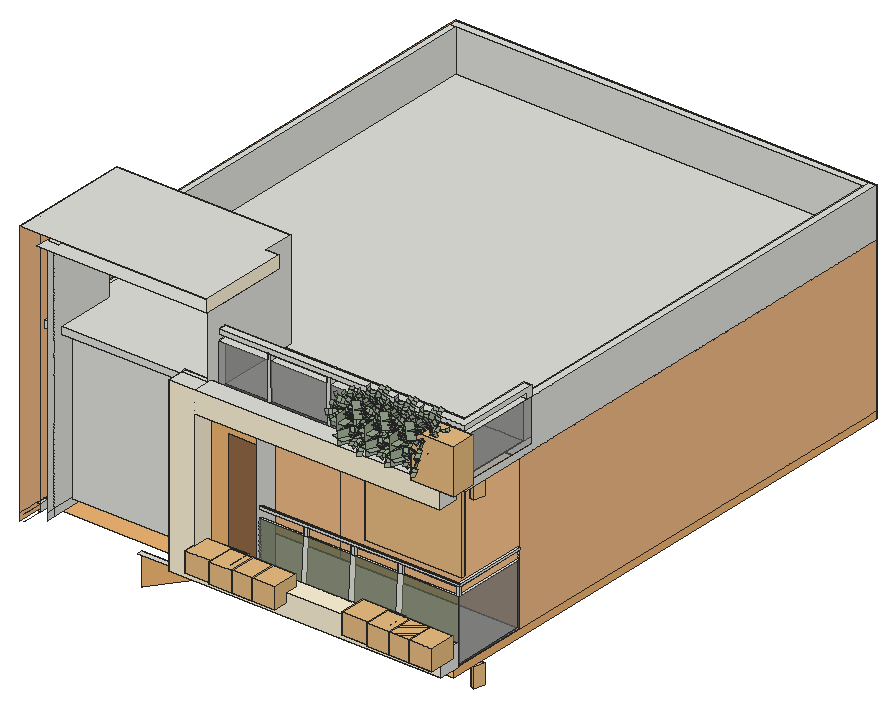
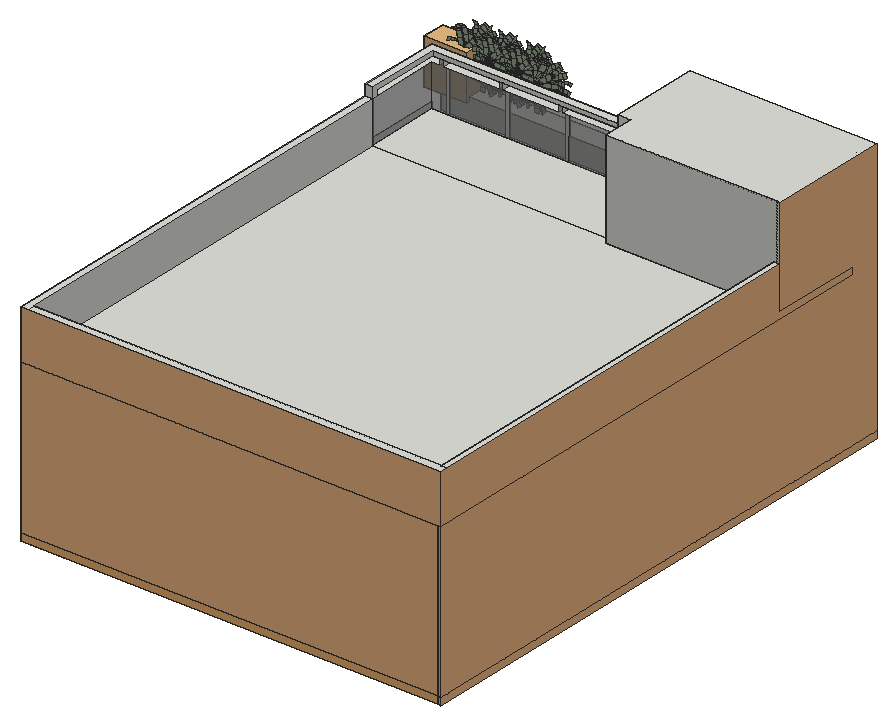
# SketchUp Ruby script. Lengths in inches.
U = 1.inch
M = Sketchup.active_model
def pt(a) = Geom::Point3d.new(a.map { |v| v * U })
def face(e, loops, mat)
  f = e.add_face(loops[0].map { |a| pt(a) })
  loops[1..].each { |l| e.add_face(l.map { |a| pt(a) }).erase! }
  f.material = f.back_material = mat if mat
  f
end
# faces: each face lists its corners as indices into pts; further lists are holes
def faces(e, pts, list, mat = nil) = list.each { |f| face(e, (f[0].is_a?(Array) ? f : [f]).map { |l| l.map { |i| pts[i] } }, mat) }
# xy, xz, yz: faces in a plane at the given z, y or x. An outline is a flat list of corners, or four numbers for a rectangle; further outlines are holes
def ring(l) = l.size == 4 ? [[l[0], l[1]], [l[2], l[1]], [l[2], l[3]], [l[0], l[3]]] : l.each_slice(2).to_a
def flat(e, list, mat, &to3) = list.each { |f| face(e, (f[0].is_a?(Array) ? f : [f]).map { |l| ring(l).map { |u, v| to3.(u, v) } }, mat) }
def xy(e, z, list, mat = nil) = flat(e, list, mat) { |x, y| [x, y, z] }
def xz(e, y, list, mat = nil) = flat(e, list, mat) { |x, z| [x, y, z] }
def yz(e, x, list, mat = nil) = flat(e, list, mat) { |y, z| [x, y, z] }
def lines(e, pts, list) = list.each { |a, b| e.add_line(pt(pts[a]), pt(pts[b])) }
# prism: a flat outline (further loops are holes) pulled along v
def prism(e, loops, v, mat = nil)
  f = face(e, loops, mat); d = Geom::Vector3d.new(v.map { |x| x * U })
  f.pushpull(f.normal.samedirection?(d) ? d.length : -d.length)
end
def box(e, o, s, mat = nil) = prism(e, [[o, [o[0] + s[0], o[1], o[2]], [o[0] + s[0], o[1] + s[1], o[2]], [o[0], o[1] + s[1], o[2]]]], [0, 0, s[2]], mat)
def at(x, y, z, deg = 0) = Geom::Transformation.translation(pt([x, y, z])) * Geom::Transformation.rotation(ORIGIN, Z_AXIS, deg.degrees)
def axes(o, x, y, z) = Geom::Transformation.new([*x, 0, *y, 0, *z, 0, *pt(o).to_a, 1])
def part(name) = M.definitions.add(name)
# library, detail: a bought-in or finely detailed component or shape, given as its bounding box
def library(name, o, s) = part(name).tap { |d| box(d.entities, o, s) }
def detail(e, o, s) = box(e.add_group.entities, o, s)
def put(e, d, t, mat = nil) = e.add_instance(d, t).tap { |i| i.material = mat if mat }
def group(e, t, mat = nil) = e.add_group.tap { |g| g.transformation = t; g.material = mat if mat }.entities
root = M.entities
M.materials.add("[Brick Antique 01]").color = [147, 105, 71]
M.materials.add("[Color C03]").color = [242, 183, 116]
M.materials.add("[Color C03]1").color = [242, 188, 135]
M.materials.add("[Color D01]").color = [255, 245, 216]
M.materials.add("[Translucent Glass Dark Green]").color = [62, 91, 5]
M.materials["[Translucent Glass Dark Green]"].alpha = 0.5
M.materials.add("[Translucent Glass Gray]").color = [128, 128, 128]
M.materials["[Translucent Glass Gray]"].alpha = 0.5
M.materials.add("hymenocallis littoralis").color = [156, 172, 146]
c1 = library("[SKP_VZ_MOD_01]_WALL_LIGHT",[-1.1,-1.22,0],[3.54,2.36,6.3])
c2 = library("Plante \#58",[-0.43,-1.58,0],[20.84,18.06,17.59])
c3 = part("Group\#4")
xy(c3.entities,35.0625,[[0,2,3.83,3.5]])
p = [[0,2,35.0625],[0,0,0],[3.83,0,0],[3.83,2,35.0625]]
faces(c3.entities,p,[[0,1,2,3]])
c4 = library("Group\#6",[0,0,0],[84,7.18,89.375])
c5 = part("Group\#856")
xy(c5.entities,7.38,[[0,0,5.5,15.91]],"hymenocallis littoralis")
p = [[5.5,28.78,0],[5.5,26.79,3.44],[0,26.79,3.44],[0,28.78,0],[0,23.75,6],[5.5,23.75,6],
  [0,15.91,7.38],[5.5,15.91,7.38]]
faces(c5.entities,p,[[0,1,2,3],[4,2,1,5],[6,4,5,7]],"hymenocallis littoralis")
c6 = part("Group\#12")
xy(c6.entities,7.38,[[0,0,5.5,15.91],[0,15.91,5.5,23.87]],"hymenocallis littoralis")
p = [[5.5,31.07,4.3],[5.5,27.74,6.47],[0,27.74,6.47],[0,31.07,4.3],[0,23.87,7.38],[5.5,23.87,7.38]]
faces(c6.entities,p,[[0,1,2,3],[4,2,1,5]],"hymenocallis littoralis")
c7 = part("Group\#857")
xy(c7.entities,7.38,[[0,0,5.6,15.91]],"hymenocallis littoralis")
p = [[5.6,28.78,0],[5.6,26.79,3.44],[0,26.79,3.44],[0,28.78,0],[0,23.75,6],[5.6,23.75,6],
  [0,15.91,7.38],[5.6,15.91,7.38]]
faces(c7.entities,p,[[0,1,2,3],[4,2,1,5],[6,4,5,7]],"hymenocallis littoralis")
c8 = part("Group\#855")
put(c8.entities,c6,axes([6.09,8.57,-0.52],[0.446,0.85617,0.26089],[-0.18444,-0.19731,0.96283],[0.87582,-0.47754,0.0699]))
put(c8.entities,c6,axes([6.29,7.28,-1.71],[0.37058,0.92707,-0.05667],[-0.32382,0.19004,0.99128],[0.87712,-0.32925,0.34964]))
put(c8.entities,c6,axes([11.04,16.14,-0.7],[1,0,0],[0,0.16628,1.02662],[0,-1.18456,0.19186]))
c9 = part("Group\#860")
put(c9.entities,c5,axes([24.57,32.05,-1.76],[0.9552,-0.22102,-0.19681],[0.4036,0.95545,0.88585],[-0.00568,-0.67859,0.7345]))
put(c9.entities,c5,axes([23.95,29.24,-2.4],[0,1,0],[-0.76041,0,0.64945],[0.64945,0,0.76041]))
put(c9.entities,c5,axes([24.22,24.72,-0.48],[-0.70711,0.70711,0],[-0.32757,-0.32757,0.80237],[0.61237,0.61237,0.5]))
put(c9.entities,c6,axes([20.66,37.22,-0.63],[1.12361,0.03262,0.39091],[-0.43499,0.29739,0.78777],[0.09852,-1.27434,0.37535]))
put(c9.entities,c5,axes([28.75,24.45,-2.4],[-1,0,0],[0,-0.76041,0.64945],[0,0.64945,0.76041]))
put(c9.entities,c7,axes([30.4,30.98,-3.7],[0.65676,-0.72002,0.22414],[0.55667,0.66341,0.5],[-0.50871,-0.20361,0.83652]))
put(c9.entities,c7,axes([32.41,29.61,-3.7],[0.04029,-0.97372,0.22414],[0.85287,0.15038,0.5],[-0.52057,0.17102,0.83652]))
put(c9.entities,c5,axes([31.89,25.85,-1.76],[-0.92056,0.33739,-0.19681],[-0.5186,-0.89824,0.88585],[0.08952,0.67268,0.7345]))
put(c9.entities,c5,axes([25.55,34.78,-0.48],[0.86603,0.5,0],[-0.25,0.43301,0.86603],[0.43301,-0.75,0.5]))
put(c9.entities,c7,axes([20.4,16.9375,-8.07],[-0.70711,0.70711,0],[-0.35754,-0.35754,0.65422],[1.3987,1.3987,1.52882]))
put(c9.entities,c5,axes([32.86,34.14,-0.48],[0.76604,-0.64279,0],[0.32139,0.38302,0.86603],[-0.55667,-0.66341,0.5]))
put(c9.entities,c5,axes([27.15,34.7,-0.1],[0.82472,-0.17528,-0.53769],[0.53769,0.53769,0.64945],[0.17528,-0.82472,0.53769]))
put(c9.entities,c5,axes([33.58,28.77,-2.4],[0,-1,0],[0.76041,0,0.64945],[-0.64945,0,0.76041]))
put(c9.entities,c5,axes([26.43,23.87,-2.81],[-0.75126,0.04415,0.65853],[0.53769,-0.53769,0.64945],[0.38276,0.84199,0.3802]))
put(c9.entities,c5,axes([28.78,23.98,-2.4],[-1,0,0],[0,-0.76041,0.64945],[0,0.64945,0.76041]))
put(c9.entities,c5,axes([25.39,25.38,-2.4],[-0.70711,0.70711,0],[-0.53769,-0.53769,0.64945],[0.45923,0.45923,0.76041]))
put(c9.entities,c5,axes([27.32,21.63,-0.1],[-0.45923,0.70711,-0.53769],[-0.76041,0,0.64945],[0.45923,0.70711,0.53769]))
put(c9.entities,c5,axes([25.17,27.625,-1.76],[0.56416,0.80187,-0.19681],[-0.66673,0.66673,0.80532],[0.62659,-0.26057,0.7345]))
put(c9.entities,c7,axes([27.59,27.04,-3.96],[-0.8993,-0.06127,0.43301],[0.2962,-0.8138,0.5],[0.32175,0.57791,0.75]))
put(c9.entities,c7,axes([26.98,24.5,-3.18],[-0.5,0.86603,0],[-0.75,-0.43301,0.5],[0.43301,0.25,0.86603]))
put(c9.entities,c7,axes([24.55,27.74,-3.7],[0.29517,0.92878,0.22414],[-0.85287,0.15038,0.5],[0.43068,-0.33875,0.83652]))
put(c9.entities,c7,axes([24.26,29.8,-3.18],[0.76604,0.64279,0],[-0.47317,0.5639,0.425],[0.32139,-0.38302,0.86603]))
put(c9.entities,c7,axes([25.98,32.46,-3.18],[1,0,0],[0,0.86603,0.5],[0,-0.5,0.86603]))
put(c9.entities,c5,axes([28.78,33.57,-2.4],[1,0,0],[0,0.76041,0.64945],[0,-0.64945,0.76041]))
put(c9.entities,c8,at(14.99,21.38,2.5))
put(c9.entities,c6,axes([34.63,26.34,-1.46],[-0.70089,-0.70877,0.07994],[0.4756,-0.38088,0.79293],[-0.53156,0.59378,0.60405]))
put(c9.entities,c6,axes([28.14,16.92,1.8125],[-1.19719,0.6912,0],[-0.09607,-0.16641,0.94244],[0.68444,1.18549,0.17613]))
put(c9.entities,c6,axes([31.5625,35.84,0.97],[0.66765,-1.1564,0.35779],[0.04445,0.30732,0.91033],[-1.20828,-0.64496,0.17012]))
put(c9.entities,c6,axes([38.94,22.51,0.89],[-0.97932,-0.67164,-0.05202],[0.27787,-0.41401,0.90999],[-0.85985,0.93577,0.32097]))
put(c9.entities,c6,axes([38.44,21.09,1.98],[-1.02864,-0.54856,0.2395],[0.33481,0.06999,0.88388],[-0.77261,1.08328,0.06417]))
put(c9.entities,c7,axes([35.02,30.51,-1.3],[-0.17365,-0.98481,0],[0.60224,-0.10619,0.79122],[-0.7792,0.13739,0.61153]))
put(c9.entities,c7,axes([29.41,22.33,-1.3],[-0.93969,0.34202,0],[-0.20915,-0.57465,0.79122],[0.27061,0.74351,0.61153]))
put(c9.entities,c6,axes([19.64,36,-1.62],[1.18194,0.09546,0.08234],[-0.14377,0.68823,0.76313],[0.21457,-1.1326,0.62386]))
put(c9.entities,c7,axes([24.25,24.14,-1.3],[-0.34202,0.93969,0],[-0.57465,-0.20915,0.79122],[0.74351,0.27061,0.61153]))
put(c9.entities,c7,axes([25.98,34.61,-1.3],[1,0,0],[0,0.61153,0.79122],[0,-0.79122,0.61153]))
put(c9.entities,c7,axes([31.16,34.41,-1.64],[0.56518,-0.80224,-0.19234],[0.73413,0.34233,0.72935],[-0.47639,-0.50772,0.71782]))
put(c9.entities,c7,axes([40.52,26.84,-5.82],[-0.42262,-0.90631,0],[0.48019,-0.22391,0.68552],[-1.43418,0.66877,1.22305]))
put(c9.entities,c5,axes([29.86,38.42,-1.01],[0.89064,-0.37013,0.26413],[-0.03924,0.63286,1.01918],[-0.45353,-0.76487,0.45748]))
put(c9.entities,c5,axes([29.34,22.4,-0.48],[-0.99619,-0.08716,0],[0.04358,-0.4981,0.86603],[-0.07548,0.86273,0.5]))
c10 = part("Group\#859")
put(c10.entities,c5,axes([24.57,32.05,-1.76],[0.9552,-0.22102,-0.19681],[0.4036,0.95545,0.88585],[-0.00568,-0.67859,0.7345]))
put(c10.entities,c5,axes([23.95,29.24,-2.4],[0,1,0],[-0.76041,0,0.64945],[0.64945,0,0.76041]))
put(c10.entities,c5,axes([24.22,24.72,-0.48],[-0.70711,0.70711,0],[-0.32757,-0.32757,0.80237],[0.61237,0.61237,0.5]))
put(c10.entities,c6,axes([22.87,39.97,-0.63],[1.12361,0.03262,0.39091],[-0.43499,0.29739,0.78777],[0.09852,-1.27434,0.37535]))
put(c10.entities,c5,axes([28.75,24.45,-2.4],[-1,0,0],[0,-0.76041,0.64945],[0,0.64945,0.76041]))
put(c10.entities,c7,axes([30.4,30.98,-3.7],[0.65676,-0.72002,0.22414],[0.55667,0.66341,0.5],[-0.50871,-0.20361,0.83652]))
put(c10.entities,c7,axes([32.41,29.61,-3.7],[0.04029,-0.97372,0.22414],[0.85287,0.15038,0.5],[-0.52057,0.17102,0.83652]))
put(c10.entities,c5,axes([31.89,25.85,-1.76],[-0.92056,0.33739,-0.19681],[-0.5186,-0.89824,0.88585],[0.08952,0.67268,0.7345]))
put(c10.entities,c5,axes([25.55,34.78,-0.48],[0.86603,0.5,0],[-0.25,0.43301,0.86603],[0.43301,-0.75,0.5]))
put(c10.entities,c7,axes([20.4,16.9375,-8.07],[-0.70711,0.70711,0],[-0.35754,-0.35754,0.65422],[1.3987,1.3987,1.52882]))
put(c10.entities,c5,axes([32.86,34.14,-0.48],[0.76604,-0.64279,0],[0.32139,0.38302,0.86603],[-0.55667,-0.66341,0.5]))
put(c10.entities,c5,axes([27.15,34.7,-0.1],[0.82472,-0.17528,-0.53769],[0.53769,0.53769,0.64945],[0.17528,-0.82472,0.53769]))
put(c10.entities,c5,axes([33.58,28.77,-2.4],[0,-1,0],[0.76041,0,0.64945],[-0.64945,0,0.76041]))
put(c10.entities,c5,axes([26.43,23.87,-2.81],[-0.75126,0.04415,0.65853],[0.53769,-0.53769,0.64945],[0.38276,0.84199,0.3802]))
put(c10.entities,c5,axes([28.78,23.98,-2.4],[-1,0,0],[0,-0.76041,0.64945],[0,0.64945,0.76041]))
put(c10.entities,c5,axes([25.39,25.38,-2.4],[-0.70711,0.70711,0],[-0.53769,-0.53769,0.64945],[0.45923,0.45923,0.76041]))
put(c10.entities,c5,axes([27.32,21.63,-0.1],[-0.45923,0.70711,-0.53769],[-0.76041,0,0.64945],[0.45923,0.70711,0.53769]))
put(c10.entities,c5,axes([25.17,27.625,-1.76],[0.56416,0.80187,-0.19681],[-0.66673,0.66673,0.80532],[0.62659,-0.26057,0.7345]))
put(c10.entities,c7,axes([27.59,27.04,-3.96],[-0.8993,-0.06127,0.43301],[0.2962,-0.8138,0.5],[0.32175,0.57791,0.75]))
put(c10.entities,c7,axes([33.07,28.9375,-1.86],[-0.5,0.86603,0],[-0.86347,-0.49852,0.1661],[0.11853,0.06843,0.98016]))
put(c10.entities,c7,axes([24.55,27.74,-3.7],[0.29517,0.92878,0.22414],[-0.85287,0.15038,0.5],[0.43068,-0.33875,0.83652]))
put(c10.entities,c7,axes([24.26,29.8,-3.18],[0.76604,0.64279,0],[-0.47317,0.5639,0.425],[0.32139,-0.38302,0.86603]))
put(c10.entities,c7,axes([25.98,32.46,-3.18],[1,0,0],[0,0.86603,0.5],[0,-0.5,0.86603]))
put(c10.entities,c5,axes([28.78,33.57,-2.4],[1,0,0],[0,0.76041,0.64945],[0,-0.64945,0.76041]))
put(c10.entities,c8,at(14.99,21.38,2.5))
put(c10.entities,c6,axes([34.63,26.34,-1.46],[-0.70089,-0.70877,0.07994],[0.4756,-0.38088,0.79293],[-0.53156,0.59378,0.60405]))
put(c10.entities,c6,axes([28.14,16.92,1.8125],[-1.19719,0.6912,0],[-0.09607,-0.16641,0.94244],[0.68444,1.18549,0.17613]))
put(c10.entities,c6,axes([31.5625,35.84,0.97],[0.66765,-1.1564,0.35779],[0.04445,0.30732,0.91033],[-1.20828,-0.64496,0.17012]))
put(c10.entities,c6,axes([38.94,22.51,0.89],[-0.97932,-0.67164,-0.05202],[0.27787,-0.41401,0.90999],[-0.85985,0.93577,0.32097]))
put(c10.entities,c6,axes([38.44,21.09,1.98],[-1.02864,-0.54856,0.2395],[0.33481,0.06999,0.88388],[-0.77261,1.08328,0.06417]))
put(c10.entities,c7,axes([35.02,30.51,-1.3],[-0.17365,-0.98481,0],[0.60224,-0.10619,0.79122],[-0.7792,0.13739,0.61153]))
put(c10.entities,c7,axes([29.41,22.33,-1.3],[-0.93969,0.34202,0],[-0.20915,-0.57465,0.79122],[0.27061,0.74351,0.61153]))
put(c10.entities,c6,axes([19.64,36,-1.62],[1.18194,0.09546,0.08234],[-0.14377,0.68823,0.76313],[0.21457,-1.1326,0.62386]))
put(c10.entities,c7,axes([24.25,24.14,-1.3],[-0.34202,0.93969,0],[-0.57465,-0.20915,0.79122],[0.74351,0.27061,0.61153]))
put(c10.entities,c7,axes([25.98,34.61,-1.3],[1,0,0],[0,0.61153,0.79122],[0,-0.79122,0.61153]))
put(c10.entities,c7,axes([31.16,34.41,-1.64],[0.56518,-0.80224,-0.19234],[0.73413,0.34233,0.72935],[-0.47639,-0.50772,0.71782]))
put(c10.entities,c7,axes([40.52,26.84,-5.82],[-0.42262,-0.90631,0],[0.48019,-0.22391,0.68552],[-1.43418,0.66877,1.22305]))
put(c10.entities,c5,axes([29.86,38.42,-1.01],[0.89064,-0.37013,0.26413],[-0.03924,0.63286,1.01918],[-0.45353,-0.76487,0.45748]))
put(c10.entities,c5,axes([29.34,22.4,-0.48],[-0.99619,-0.08716,0],[0.04358,-0.4981,0.86603],[-0.07548,0.86273,0.5]))
put(c10.entities,c7,axes([25.22,28.39,-0.16],[0.48481,0.87462,0],[-0.87203,0.48338,0.1661],[0.11971,-0.06635,0.98016]))
put(c10.entities,c7,axes([24.56,24.29,-4.78],[0.48481,0.87462,0],[-0.87203,0.48338,0.1661],[0.11971,-0.06635,0.98016]))
put(c10.entities,c7,axes([23.9375,27.06,-4.78],[0.99753,0.07018,0],[-0.06998,0.99459,0.1661],[0.00961,-0.13653,0.98016]))
put(c10.entities,c7,axes([25.92,29.09,-4.78],[0.6025,-0.79812,0],[0.79576,0.60072,0.1661],[-0.10924,-0.08246,0.98016]))
put(c10.entities,c7,axes([28.7,28.53,-4.78],[-0.34082,-0.94013,0],[0.93735,-0.33981,0.1661],[-0.12867,0.04665,0.98016]))
c11 = part("Group\#858")
xz(c11.entities,10.07,[[9.07,0,10.07,31.01],[0,31.01,0,45.12,20.13,45.12,20.13,31.01,10.07,31.01,10.07,32.58,9.07,32.58,9.07,31.01]],"hymenocallis littoralis")
yz(c11.entities,10.07,[[0,31.01,20.13,45.12]],"hymenocallis littoralis")
p = [[9.57,9.2,0],[10.07,10.07,0],[10.07,10.07,31.01],[10.07,10.07,32.58],[9.57,9.2,32.58]]
faces(c11.entities,p,[[0,1,2,3,4]],"hymenocallis littoralis")
c12 = part("cây lá nắng")
put(c12.entities,c9,axes([49.26,-2.75,0],[0.63109,0.63109,0],[-0.63109,0.63109,0],[0,0,0.935]))
put(c12.entities,c10,axes([26.6,-8.68,0],[0.63109,0.63109,0],[-0.63109,0.63109,0],[0,0,0.935]))
put(c12.entities,c11,axes([29.71,14.29,6.94],[0.425,0.73612,0],[-0.6771,0.39092,-0.33349],[-0.26859,0.15507,0.72712]))
put(c12.entities,c11,axes([42.0625,26.12,6.94],[0.85,0,0],[0,0.78185,-0.33349],[0,0.33349,0.78185]))
put(c12.entities,c9,axes([7.3125,23.0625,0],[0.8925,0,0],[0,0.8925,0],[0,0,0.935]))
put(c12.entities,c11,axes([24.4375,40.23,2.05],[0.85,0,0],[0,0.85,0],[0,0,0.85]))
c13 = part("Planting+101")
put(c13.entities,c12,axes([21.34,32.96,-4.59],[0,-0.71,0],[-0.71,0,0],[0,0,0.71]))
xy(root,114,[[196.3125,117.47,241.3125,128.9],[280.3125,117.47,364.3125,146.78]])
xy(root,138,[[139.52,45.9,196.3125,50.65],[196.3125,45.9,199.52,50.65],[49.3125,49.9,52.3125,59.47],[196.3125,50.65,199.52,59.47],[49.3125,59.47,52.3125,109.47],
  [49.3125,109.47,52.3125,117.47],[49.3125,117.47,52.3125,501.47],[52.3125,117.47,412.3125,501.47]])
xy(root,138,[[199.52,45.9,199.52,59.47,196.3125,59.47,196.3125,117.47,256.62,117.47,256.62,45.9],[[256.62,45.9,412.3125,117.47],[399.28,70.78,410.47,80.47]],[52.3125,59.47,196.3125,117.47]],"[Color C03]")
xy(root,144,[[177.125,31.9,412.3125,45.9],[177.125,45.9,199.52,49.9],[199.52,45.9,239.27,49.9],[239.27,45.9,412.3125,49.9],[49.3125,49.9,52.3125,57.47],
  [239.27,49.9,412.3125,51.9],[239.27,51.9,412.3125,53.4],[239.27,53.4,410.25,53.4,410.25,117.47,52.3125,117.47,52.3125,68.97,239.27,68.97],[410.25,53.4,412.3125,117.47],[49.3125,57.47,52.3125,109.47],
  [49.3125,109.47,52.3125,117.47],[49.3125,117.47,52.3125,501.47],[52.3125,117.47,412.3125,501.47]])
xy(root,162.75,[[199.52,31.9,412.3125,49.9]],"[Color D01]")
xy(root,168,[[280.3125,117.47,364.3125,133.97]])
xy(root,197.8125,[[239.27,51.9,277.74,53.4],[277.74,51.9,281.49,53.4],[281.49,51.9,281.57,53.4],[281.57,51.9,318.55,53.4],[318.55,51.9,322.38,53.4],
  [322.38,51.9,359.36,53.4],[359.36,51.9,363.19,53.4],[363.19,51.9,410.25,53.4],[410.25,53.53,412.3125,117.47]])
xy(root,205,[[239.27,51.9,277.74,53.4],[277.74,51.9,281.49,53.4],[281.49,51.9,318.55,53.4],[318.55,51.9,322.38,53.4],[322.38,51.9,359.36,53.4],
  [359.36,51.9,363.19,53.4],[363.19,51.9,410.25,53.4],[410.25,53.53,412.3125,117.47]])
xy(root,207,[[239.27,51.9,412.3125,53.4],[410.25,53.4,412.3125,117.47]])
xy(root,252,[[280.3125,117.47,364.3125,133.97]])
xy(root,273.03,[[199.52,31.9,410.875,49.9]],"[Color D01]")
xy(root,276,[[199.52,49.9,239.27,57.47],[49.3125,57.47,52.3125,68.97],[52.3125,57.47,196.3125,68.97],[196.3125,57.47,196.3125,68.97,239.27,68.97,239.27,57.9,199.52,57.9,199.52,57.47],[199.52,57.47,239.27,57.9],
  [49.3125,68.97,52.3125,109.47],[52.3125,68.97,196.3125,117.47],[49.3125,109.47,52.3125,117.47],[49.3125,117.47,52.3125,501.47]])
xy(root,276,[[239.27,57.9,239.27,68.97,196.3125,68.97,196.3125,117.47,256.62,117.47,256.62,57.9],[256.62,57.9,412.3125,117.47]],"[Color D01]")
xy(root,282,[[49.3125,57.47,52.3125,135.65],[52.3125,57.47,196.3125,135.65],[196.3125,57.47,199.52,129.47],[199.52,65.22,405.9375,129.47],[199.52,129.47,405.9375,129.47,405.9375,494.53,54.75,494.53,54.75,135.65,199.52,135.65],
  [196.3125,129.47,199.52,135.65]])
xy(root,291.78,[[177.125,31.9,199.52,45.9],[199.52,31.9,410.875,49.9],[177.125,45.9,199.52,49.9]])
xy(root,318.4375,[[199.52,57.9,241.8125,65.22],[244.9375,57.9,293.25,65.22],[296.375,57.9,344.6875,65.22],[347.8125,57.9,396.125,65.22],[399.25,57.9,412.3125,57.9,412.3125,124.88,405.9375,124.88,405.9375,65.22,399.25,65.22],
  [405.78,124.88,405.9375,129.47],[405.9375,124.88,412.3125,129.47],[405.9375,129.47,412.3125,501.47],[49.3125,135.65,54.75,494.53],[49.3125,494.53,405.9375,501.47]])
xy(root,323.625,[[199.52,57.9,241.8125,65.22],[241.8125,57.9,244.9375,65.22],[244.9375,57.9,293.25,65.22],[293.25,57.9,296.375,65.22],[296.375,57.9,344.6875,65.22],
  [344.6875,57.9,347.8125,65.22],[347.8125,57.9,396.125,65.22],[396.125,57.9,399.25,65.22],[399.25,57.9,399.25,65.22,405.78,65.22,405.78,124.88,412.3125,124.88,412.3125,57.9]])
xy(root,327.3125,[[199.52,57.9,412.3125,57.9,412.3125,129.47,405.78,129.47,405.78,65.22,199.52,65.22]])
xy(root,354.99,[[63.88,31.9,63.88,42.9,73.88,42.9,73.88,45.9,210.46,45.9,210.46,31.9],[63.88,42.9,63.88,49.9,199.52,49.9,199.52,45.9,73.88,45.9,73.88,42.9],[199.52,45.9,210.46,49.9],[63.88,49.9,199.52,109.47],[199.52,49.9,210.46,109.47]])
xy(root,366,[[49.3125,31.9,210.46,31.9,210.46,109.47,199.52,109.47,199.52,135.65,49.3125,135.65]])
xz(root,31.9,[[177.125,144,412.3125,144,412.3125,162.75,199.52,162.75,199.52,273.03,410.875,273.03,410.875,291.78,177.125,291.78]],"[Color D01]")
xz(root,49.9,[[177.125,144,177.125,291.78,199.52,291.78,199.52,276,239.27,276,239.27,273.03,199.52,273.03,199.52,162.75,239.27,162.75,239.27,144],[239.27,144,412.3125,162.75],[239.27,273.03,239.27,276,199.52,276,199.52,291.78,410.875,291.78,410.875,273.03]])
xz(root,49.9,[[214.22,162.75,239.27,255.4]],"[Brick Antique 01]")
xz(root,49.9,[[199.52,162.75,214.22,162.75,214.22,255.4,239.27,255.4,239.27,273.03,199.52,273.03]],"[Color C03]")
xz(root,50.65,[[139.52,109.96,199.52,138,139.52,138]],"[Color C03]")
xz(root,51.9,[[277.74,197.8125,281.49,205],[318.55,197.8125,322.38,205],[359.36,197.8125,363.19,205],[410.25,197.8125,412.3125,205],[239.27,205,412.3125,207]])
xz(root,51.9,[[239.27,144,412.3125,197.8125]],"[Translucent Glass Gray]")
xz(root,53.4,[[277.74,197.8125,281.49,205],[318.55,197.8125,322.38,205],[359.36,197.8125,363.19,205],[239.27,205,410.25,207]])
xz(root,53.4,[[239.27,144,410.25,197.8125]],"[Translucent Glass Dark Green]")
xz(root,53.53,[[410.25,197.8125,412.3125,205]])
xz(root,57.47,[[49.3125,276,52.3125,282],[52.3125,276,196.3125,282],[196.3125,276,199.52,282]])
xz(root,57.9,[[242.04,276,245.16,276,244.9375,318.4375,244.9375,323.625,241.8125,323.625,241.8125,318.4375],[293.47,276,296.6,276,296.375,318.4375,296.375,323.625,293.25,323.625,293.25,318.4375],[344.91,276,348.04,276,347.8125,318.4375,347.8125,323.625,344.6875,323.625,344.6875,318.4375],[396.35,276,399.47,276,399.25,318.4375,399.25,323.625,396.125,323.625,396.125,318.4375],[199.52,323.625,412.3125,327.3125]])
xz(root,57.9,[[199.52,276,242.04,276,241.8125,318.4375,199.52,318.4375],[245.16,276,293.47,276,293.25,318.4375,244.9375,318.4375],[296.6,276,344.91,276,344.6875,318.4375,296.375,318.4375],[348.04,276,396.35,276,396.125,318.4375,347.8125,318.4375],[399.47,276,412.3125,276,412.3125,318.4375,399.25,318.4375]],"[Translucent Glass Gray]")
xz(root,65.22,[[199.52,323.625,405.78,327.3125]])
xz(root,65.22,[[199.52,282,199.52,318.4375,241.8125,318.4375,241.8125,323.625,244.9375,323.625,244.9375,318.4375,293.25,318.4375,293.25,323.625,296.375,323.625,296.375,318.4375,344.6875,318.4375,344.6875,323.625,347.8125,323.625,347.8125,318.4375,396.125,318.4375,396.125,323.625,399.25,323.625,399.25,318.4375,405.9375,318.4375,405.9375,282]],"[Translucent Glass Gray]")
xz(root,68.97,[[52.3125,144,239.27,276]])
xz(root,109.47,[[199.52,354.99,210.46,366]])
xz(root,117.47,[[52.3125,144,196.3125,276],[410.25,197.8125,412.3125,205]])
xz(root,117.47,[[196.3125,144,256.62,276],[[256.62,144,410.25,144,410.25,207,412.3125,207,412.3125,276,256.62,276],[280.3125,168,364.3125,252]]],"[Color C03]1")
xz(root,124.88,[[405.78,318.4375,412.3125,323.625]])
xz(root,129.47,[[405.78,318.4375,412.3125,327.3125]])
xz(root,133.97,[[280.3125,168,364.3125,252]])
xz(root,135.65,[[49.3125,282,52.3125,318.4375],[52.3125,282,54.75,318.4375],[54.75,282,54.75,318.4375,52.3125,318.4375,52.3125,366,199.52,366,199.52,282],[49.3125,318.4375,52.3125,366]])
xz(root,494.53,[[54.75,282,405.9375,318.4375]])
xz(root,501.47,[[49.3125,138,52.3125,144],[52.3125,138,412.3125,144],[49.3125,144,52.3125,276]],"[Color C03]")
xz(root,501.47,[[52.3125,144,412.3125,276],[49.3125,276,412.3125,318.4375]],"[Color C03]1")
yz(root,49.3125,[[31.9,138,501.47,144],[31.9,144,31.9,366,135.65,366,135.65,282,57.47,282,57.47,276,501.47,276,501.47,144],[57.47,276,57.47,282,135.65,282,135.65,318.4375,501.47,318.4375,501.47,276]],"[Color C03]1")
yz(root,52.3125,[[49.9,138,109.47,144],[109.47,138,501.47,144],[68.97,144,109.47,276],[109.47,144,117.47,276],[117.47,144,501.47,276]])
yz(root,54.75,[[135.65,282,494.53,318.4375]])
yz(root,63.88,[[42.9,138,49.9,144],[49.9,138,109.47,144],[42.9,144,49.9,354.99],[49.9,144,109.47,354.99]])
yz(root,177.125,[[31.9,144,45.9,291.78],[45.9,144,49.9,291.78]])
yz(root,199.52,[[49.9,276,57.47,282],[57.47,276,57.9,282],[[49.9,282,57.9,282,57.9,318.4375,65.22,318.4375,65.22,282,135.65,282,135.65,366,109.47,366,109.47,354.99,45.9,354.99,45.9,291.78,49.9,291.78],[57.9,323.625,65.22,327.3125]],[57.9,282,65.22,318.4375],[57.9,323.625,65.22,327.3125]])
yz(root,199.52,[[31.9,162.75,49.9,273.03]],"[Color D01]")
yz(root,210.46,[[31.9,354.99,109.47,366]],"[Color D01]")
yz(root,239.27,[[[49.9,144,51.9,144,51.9,197.8125,53.4,197.8125,53.4,144,68.97,144,68.97,276,49.9,276],[51.9,205,53.4,207]],[51.9,144,53.4,197.8125],[51.9,205,53.4,207]])
yz(root,241.8125,[[57.9,318.4375,65.22,323.625]])
yz(root,244.9375,[[57.9,318.4375,65.22,323.625]])
yz(root,277.74,[[51.9,197.8125,53.4,205]])
yz(root,280.3125,[[117.47,168,133.97,252]])
yz(root,281.49,[[51.9,197.8125,53.4,205]])
yz(root,293.25,[[57.9,318.4375,65.22,323.625]])
yz(root,296.375,[[57.9,318.4375,65.22,323.625]])
yz(root,318.55,[[51.9,197.8125,53.4,205]])
yz(root,322.38,[[51.9,197.8125,53.4,205]])
yz(root,344.6875,[[57.9,318.4375,65.22,323.625]])
yz(root,347.8125,[[57.9,318.4375,65.22,323.625]])
yz(root,359.36,[[51.9,197.8125,53.4,205]])
yz(root,363.19,[[51.9,197.8125,53.4,205]])
yz(root,364.3125,[[117.47,168,133.97,252]])
yz(root,396.125,[[57.9,318.4375,65.22,323.625]])
yz(root,399.25,[[57.9,318.4375,65.22,323.625]])
yz(root,405.78,[[124.88,318.4375,124.88,323.625,65.22,323.625,65.22,327.3125,129.47,327.3125,129.47,318.4375]])
yz(root,405.9375,[[129.47,282,494.53,318.4375]])
yz(root,405.9375,[[65.22,282,129.47,318.4375]],"[Translucent Glass Gray]")
yz(root,410.25,[[53.4,144,53.4,197.8125,51.9,197.8125,51.9,205,53.4,205,53.4,207,117.47,207,117.47,205,53.53,205,53.53,197.8125,117.47,197.8125,117.47,144]],"[Translucent Glass Gray]")
yz(root,410.875,[[31.9,273.03,49.9,291.78]])
yz(root,412.3125,[[31.9,144,49.9,162.75],[51.9,197.8125,53.53,205],[51.9,205,117.47,207],[57.9,276,501.47,276,501.47,318.4375,129.47,318.4375,129.47,282,57.9,282],[124.88,318.4375,129.47,318.4375,129.47,327.3125,57.9,327.3125,57.9,323.625,124.88,323.625]])
yz(root,412.3125,[[45.9,138,501.47,144]],"[Color C03]")
yz(root,412.3125,[[117.47,144,501.47,276]],"[Color C03]1")
yz(root,412.3125,[[51.9,144,117.47,197.8125],[57.9,282,129.47,318.4375]],"[Translucent Glass Gray]")
p = [[199.52,59.47,138],[199.52,50.65,138],[139.52,50.65,109.96],[139.52,59.47,109.96],[196.3125,129.47,282],[196.25,129.47,282],
  [199.52,49.9,282],[199.52,31.9,282],[199.52,49.9,276],[199.52,31.9,276],[199.52,49.9,152.97],[199.52,31.9,152.97],
  [199.52,49.9,146.97],[199.52,31.9,146.97],[52.3125,31.9,138],[52.3125,49.9,138],[52.3125,31.9,144],[52.3125,49.9,144],
  [52.3125,49.9,366],[199.52,65.22,318.4375],[199.52,65.22,323.625]]
faces(root,p,[[0,1,2,3]],"[Color C03]")
lines(root,p,[[4,5],[6,7],[8,9],[10,11],[12,13],[14,15],[16,17],[18,17],[19,20]])
put(root,c1,axes([378.13,111.95,90.36],[0.67293,2.51141,0],[-1.55707,0.41722,0],[0,0,2.6]))
put(root,c1,axes([264.63,111.97,90.36],[0.67293,2.51141,0],[-1.50684,0.40376,0],[0,0,2.6]))
put(root,c2,axes([199.62,24.56,153.89],[1.77,0,0],[0,1.2687,0],[0,0,1]))
put(root,c2,axes([335.18,24.56,153.89],[1.77,0,0],[0,1.2687,0],[0,0,1]))
put(root,c2,axes([222.66,22.03,154.56],[1.77,0,0],[0,1.2687,0],[0,0,1]))
put(root,c2,axes([242.16,22.03,154.56],[1.77,0,0],[0,1.2687,0],[0,0,1]))
put(root,c2,axes([358.22,22.03,154.56],[1.77,0,0],[0,1.2687,0],[0,0,1]))
put(root,c2,axes([377.72,22.03,154.56],[1.77,0,0],[0,1.2687,0],[0,0,1]))
put(root,c3,at(318.55,49.9,162.75))
put(root,c3,at(359.36,49.9,162.75))
put(root,c3,at(277.74,49.9,162.75))
put(root,c4,axes([280.3125,114.23,168],[1,0,0],[0,1,0],[0,0,0.93986]))
put(root,c1,axes([264.32,112.05,235.92],[0.67293,2.51141,0],[-1.23059,0.32974,0],[0,0,2.6]))
put(root,c1,axes([377.59,111.91,235.92],[0.67293,2.51141,0],[-1.68264,0.45086,0],[0,0,2.6]))
put(root,c13,axes([345.24,43.82,308.5],[1,0,0],[0,0,1],[0,-1,0]))
put(root,c13,axes([369.49,43.82,308.5],[1,0,0],[0,0,1],[0,-1,0]))
put(root,c13,axes([391.42,43.82,308.5],[1,0,0],[0,0,1],[0,-1,0]))
put(root,c2,axes([387.41,33.68,287.81],[1.77,0,0],[0,1.12767,0],[0,0,2.21]))
